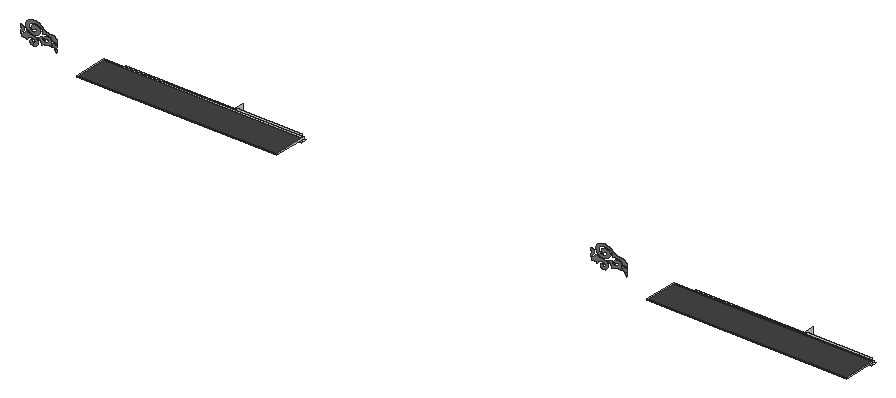
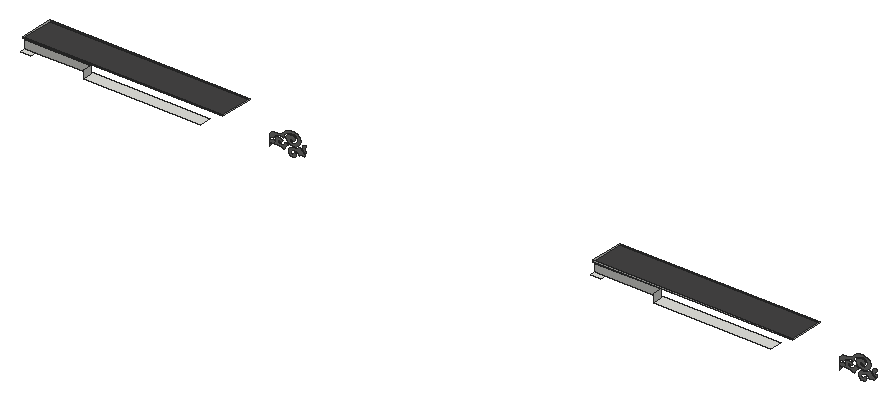
# SketchUp Ruby script. Lengths in inches.
U = 1.inch
M = Sketchup.active_model
def pt(a) = Geom::Point3d.new(a.map { |v| v * U })
def face(e, loops, mat)
  f = e.add_face(loops[0].map { |a| pt(a) })
  loops[1..].each { |l| e.add_face(l.map { |a| pt(a) }).erase! }
  f.material = f.back_material = mat if mat
  f
end
# faces: each face lists its corners as indices into pts; further lists are holes
def faces(e, pts, list, mat = nil) = list.each { |f| face(e, (f[0].is_a?(Array) ? f : [f]).map { |l| l.map { |i| pts[i] } }, mat) }
# xy, xz, yz: faces in a plane at the given z, y or x. An outline is a flat list of corners, or four numbers for a rectangle; further outlines are holes
def ring(l) = l.size == 4 ? [[l[0], l[1]], [l[2], l[1]], [l[2], l[3]], [l[0], l[3]]] : l.each_slice(2).to_a
def flat(e, list, mat, &to3) = list.each { |f| face(e, (f[0].is_a?(Array) ? f : [f]).map { |l| ring(l).map { |u, v| to3.(u, v) } }, mat) }
def xy(e, z, list, mat = nil) = flat(e, list, mat) { |x, y| [x, y, z] }
def xz(e, y, list, mat = nil) = flat(e, list, mat) { |x, z| [x, y, z] }
def yz(e, x, list, mat = nil) = flat(e, list, mat) { |y, z| [x, y, z] }
def lines(e, pts, list) = list.each { |a, b| e.add_line(pt(pts[a]), pt(pts[b])) }
# prism: a flat outline (further loops are holes) pulled along v
def prism(e, loops, v, mat = nil)
  f = face(e, loops, mat); d = Geom::Vector3d.new(v.map { |x| x * U })
  f.pushpull(f.normal.samedirection?(d) ? d.length : -d.length)
end
def box(e, o, s, mat = nil) = prism(e, [[o, [o[0] + s[0], o[1], o[2]], [o[0] + s[0], o[1] + s[1], o[2]], [o[0], o[1] + s[1], o[2]]]], [0, 0, s[2]], mat)
def at(x, y, z, deg = 0) = Geom::Transformation.translation(pt([x, y, z])) * Geom::Transformation.rotation(ORIGIN, Z_AXIS, deg.degrees)
def axes(o, x, y, z) = Geom::Transformation.new([*x, 0, *y, 0, *z, 0, *pt(o).to_a, 1])
def part(name) = M.definitions.add(name)
# library, detail: a bought-in or finely detailed component or shape, given as its bounding box
def library(name, o, s) = part(name).tap { |d| box(d.entities, o, s) }
def detail(e, o, s) = box(e.add_group.entities, o, s)
def put(e, d, t, mat = nil) = e.add_instance(d, t).tap { |i| i.material = mat if mat }
def group(e, t, mat = nil) = e.add_group.tap { |g| g.transformation = t; g.material = mat if mat }.entities
root = M.entities
M.materials.add("[0043_SaddleBrown]4").color = [124, 123, 122]
M.materials.add("[Granite Dark Gray]").color = [69, 68, 68]
xy(root,251.46,[[3079.62,589.17,3079.62,616,3336.64,616,3336.64,595.44,3457.61,595.44,3457.61,589.17],[4330.25,589.17,4330.25,616,4587.26,616,4587.26,595.44,4708.23,595.44,4708.23,589.17],[3457.61,595.44,3480.67,608.75],[4708.23,595.44,4731.3,608.75]])
xy(root,265.8125,[[3053.01,515.0625,3491.44,589.17],[4303.63,515.0625,4742.06,589.17]],"[Granite Dark Gray]")
xz(root,515.0625,[[3053.01,265.8125,3491.44,268.4375],[4303.63,265.8125,4742.06,268.4375]],"[Granite Dark Gray]")
xz(root,589.17,[[3053.01,265.8125,3491.44,268.4375],[4303.63,265.8125,4742.06,268.4375]])
xz(root,589.17,[[2899.09,240.53,2897.49,240.59,2895.9375,240.89,2894.51,241.42,2893.27,242.16,2892.27,243.07,2891.56,244.1,2891.16,245.23,2891.11,246.39,2891.17,246.75,2891.28,247.1,2891.44,247.44,2891.65,247.77,2891.91,248.09,2892.21,248.38,2892.55,248.64,2892.92,248.89,2893.33,249.1,2893.77,249.28,2894.23,249.43,2894.71,249.54,2894.79,249.03,2894.91,248.52,2895.07,248.02,2895.28,247.53,2895.52,247.05,2895.8,246.58,2896.12,246.12,2896.48,245.67,2896.87,245.24,2897.29,244.83,2897.75,244.4375,2898.24,244.07,2899.17,244.4,2900.02,244.84,2900.77,245.37,2901.4,245.97,2901.89,246.64,2902.23,247.35,2902.42,248.09,2902.44,248.85,2902.3,249.59,2902.01,250.32,2901.57,251,2900.98,251.625,2900.14,252.57,2899.07,253.38,2897.82,254.04,2896.42,254.51,2894.92,254.8,2893.37,254.88,2891.83,254.75,2890.34,254.42,2888.97,253.9,2887.76,253.2,2886.74,252.35,2885.96,251.39,2885.74,251.13,2885.54,250.86,2885.35,250.6,2885.17,250.32,2885,250.05,2884.85,249.77,2884.71,249.48,2884.58,249.2,2884.36,248.62,2884.27,248.32,2884.2,248.02,2883.51,248.6875,2882.71,249.28,2881.81,249.8,2880.83,250.24,2879.78,250.58,2878.6875,250.83,2877.55,250.97,2876.41,251.02,2875.26,250.96,2874.13,250.8,2873.04,250.54,2872,250.18,2872.22,250.49,2872.41,250.81,2872.57,251.13,2872.71,251.47,2872.83,251.8,2872.91,252.14,2872.97,252.49,2873,252.83,2873.01,253.18,2872.98,253.53,2872.93,253.875,2872.85,254.22,2874,254.84,2875.09,255.51,2876.15,256.21,2877.15,256.95,2878.11,257.73,2879.01,258.53,2879.86,259.37,2880.65,260.23,2881.38,261.12,2882.05,262.04,2882.66,262.97,2883.21,263.93,2883.82,263.15,2884.54,262.41,2885.35,261.73,2886.26,261.12,2887.25,260.57,2888.3125,260.1,2889.44,259.71,2890.61,259.41,2891.82,259.19,2893.05,259.0625,2894.29,259.03,2895.54,259.08,2897.95,258.68,2900.24,257.98,2902.32,257,2904.125,255.77,2905.61,254.34,2906.73,252.74,2907.44,251.03,2907.73,249.25,2907.58,247.46,2907.01,245.72,2906.02,244.08,2904.65,242.59,2903.52,241.76,2902.18,241.125,2900.68,240.71],[4149.72,240.53,4148.11,240.59,4146.5625,240.89,4145.14,241.42,4143.89,242.16,4142.9,243.07,4142.18,244.1,4141.79,245.23,4141.73,246.39,4141.79,246.75,4141.9,247.1,4142.07,247.44,4142.28,247.77,4142.53,248.09,4142.83,248.38,4143.17,248.64,4143.55,248.89,4143.96,249.1,4144.39,249.28,4144.85,249.43,4145.33,249.54,4145.41,249.03,4145.54,248.52,4145.7,248.02,4145.9,247.53,4146.15,247.05,4146.43,246.58,4146.75,246.12,4147.1,245.67,4147.49,245.24,4147.92,244.83,4148.375,244.4375,4148.86,244.07,4149.8,244.4,4150.65,244.84,4151.4,245.37,4152.02,245.97,4152.51,246.64,4152.86,247.35,4153.04,248.09,4153.07,248.85,4152.93,249.59,4152.64,250.32,4152.19,251,4151.6,251.625,4150.77,252.57,4149.7,253.38,4148.44,254.04,4147.04,254.51,4145.54,254.8,4143.99,254.88,4142.45,254.75,4140.97,254.42,4139.6,253.9,4138.38,253.2,4137.37,252.35,4136.58,251.39,4136.37,251.13,4136.17,250.86,4135.97,250.6,4135.79,250.32,4135.63,250.05,4135.47,249.77,4135.33,249.48,4135.21,249.2,4135.09,248.91,4134.99,248.62,4134.9,248.32,4134.83,248.02,4134.13,248.6875,4133.33,249.28,4132.44,249.8,4131.46,250.24,4130.41,250.58,4129.3125,250.83,4128.18,250.97,4127.03,251.02,4125.88,250.96,4124.75,250.8,4123.66,250.54,4122.625,250.18,4122.84,250.49,4123.03,250.81,4123.2,251.13,4123.34,251.47,4123.45,251.8,4123.54,252.14,4123.6,252.49,4123.63,252.83,4123.63,253.18,4123.61,253.53,4123.56,253.875,4123.48,254.22,4124.62,254.84,4125.72,255.51,4126.77,256.21,4127.78,256.95,4128.73,257.73,4129.63,258.53,4130.48,259.37,4131.27,260.23,4132.01,261.12,4132.68,262.04,4133.29,262.97,4133.84,263.93,4134.45,263.15,4135.16,262.41,4135.98,261.73,4136.89,261.12,4137.875,260.57,4138.9375,260.1,4140.06,259.71,4141.23,259.41,4142.44,259.19,4143.67,259.0625,4144.92,259.03,4146.16,259.08,4148.58,258.68,4150.86,257.98,4152.94,257,4154.75,255.77,4156.24,254.34,4157.35,252.74,4158.07,251.03,4158.35,249.25,4158.21,247.46,4157.63,245.72,4156.64,244.08,4155.27,242.59,4154.15,241.76,4152.8,241.125,4151.31,240.71],[2949.62,243.61,2949.34,244.05,2949.04,244.49,2948.74,244.92,2948.42,245.34,2948.09,245.77,2947.75,246.18,2947.4,246.6,2947.04,247,2946.28,247.8,2945.88,248.1875,2945.47,248.57,2945.75,248.76,2946.04,248.9375,2946.35,249.1,2946.68,249.24,2947.02,249.36,2947.37,249.47,2947.73,249.56,2948.1,249.625,2948.47,249.68,2948.85,249.71,2949.23,249.72,2949.62,249.7],[4200.24,243.61,4199.96,244.05,4199.67,244.49,4199.36,244.92,4199.05,245.34,4198.72,245.77,4198.38,246.18,4198.03,246.6,4197.29,247.4,4196.9,247.8,4196.5,248.1875,4196.1,248.57,4196.37,248.76,4196.67,248.9375,4196.98,249.1,4197.3,249.24,4197.64,249.36,4197.99,249.47,4198.35,249.56,4198.72,249.625,4199.1,249.68,4199.48,249.71,4199.86,249.72,4200.24,249.7],[2916.57,248.92,2916.46,249.99,2916.23,251.04,2915.89,252.09,2915.44,253.11,2914.89,254.1,2914.24,255.07,2913.49,255.99,2912.64,256.87,2911.71,257.7,2910.6875,258.48,2909.59,259.21,2908.42,259.87,2909.04,260.07,2910.26,260.51,2910.86,260.74,2911.45,260.97,2912.04,261.22,2912.62,261.48,2913.19,261.74,2913.75,262.01,2914.3125,262.29,2914.86,262.58,2915.4,262.88,2915.51,261.48,2916.03,260.125,2916.95,258.89,2918.23,257.82,2919.79,256.98,2921.57,256.41,2923.47,256.13,2925.42,256.15,2927.32,256.48,2929.07,257.1,2930.59,257.97,2931.81,259.07,2931.85,259.41,2931.87,259.75,2931.87,260.43,2931.81,261.11,2931.76,261.45,2931.69,261.79,2931.61,262.12,2931.52,262.46,2931.42,262.79,2931.29,263.12,2930.7,263.3,2930.07,263.42,2929.43,263.46,2928.78,263.43,2928.15,263.32,2927.55,263.15,2927,262.9,2926.5,262.6,2926.08,262.24,2925.75,261.85,2925.5,261.41,2925.36,260.96,2924.95,261.08,2924.5625,261.23,2924.18,261.39,2923.82,261.57,2923.47,261.77,2923.14,261.98,2922.83,262.2,2922.53,262.44,2922.26,262.69,2922.02,262.96,2921.79,263.23,2921.59,263.51,2922.18,264.63,2923.07,265.64,2924.23,266.5,2925.61,267.17,2927.14,267.62,2928.78,267.84,2930.4375,267.81,2932.06,267.54,2933.5625,267.03,2934.89,266.3125,2935.99,265.42,2936.81,264.375,2936.25,263.4375,2935.8,262.46,2935.48,261.47,2935.28,260.45,2935.2,259.43,2935.25,258.41,2935.43,257.39,2935.73,256.39,2936.15,255.41,2936.69,254.47,2937.35,253.56,2938.11,252.69,2936.23,252.81,2934.35,252.84,2932.46,252.8,2930.59,252.67,2928.72,252.47,2926.88,252.1875,2925.06,251.83,2923.27,251.39,2921.53,250.88,2919.82,250.3,2918.17,249.64],
  [4167.2,248.92,4167.08,249.99,4166.85,251.04,4166.51,252.09,4166.07,253.11,4165.51,254.1,4164.86,255.07,4164.11,255.99,4163.27,256.87,4162.33,257.7,4161.3125,258.48,4160.22,259.21,4159.05,259.87,4159.67,260.07,4160.89,260.51,4161.48,260.74,4162.08,260.97,4162.66,261.22,4163.24,261.48,4163.81,261.74,4164.38,262.01,4164.9375,262.29,4165.48,262.58,4166.02,262.88,4166.13,261.48,4166.66,260.125,4167.58,258.89,4168.85,257.82,4170.41,256.98,4172.19,256.41,4174.1,256.13,4176.05,256.15,4177.94,256.48,4179.69,257.1,4181.21,257.97,4182.43,259.07,4182.47,259.41,4182.49,259.75,4182.5,260.09,4182.49,260.43,4182.47,260.77,4182.43,261.11,4182.38,261.45,4182.32,261.79,4182.24,262.12,4182.15,262.46,4182.04,262.79,4181.92,263.12,4181.33,263.3,4180.7,263.42,4180.05,263.46,4179.41,263.43,4178.77,263.32,4178.17,263.15,4177.62,262.9,4177.13,262.6,4176.71,262.24,4176.37,261.85,4176.13,261.41,4175.98,260.96,4175.58,261.08,4175.1875,261.23,4174.81,261.39,4174.44,261.57,4174.09,261.77,4173.76,261.98,4173.45,262.2,4173.16,262.44,4172.89,262.69,4172.64,262.96,4172.42,263.23,4172.22,263.51,4172.8,264.63,4173.69,265.64,4174.85,266.5,4176.23,267.17,4177.77,267.62,4179.4,267.84,4181.0625,267.81,4182.68,267.54,4184.1875,267.03,4185.52,266.3125,4186.62,265.42,4187.44,264.375,4186.875,263.4375,4186.43,262.46,4186.11,261.47,4185.9,260.45,4185.83,259.43,4185.88,258.41,4186.06,257.39,4186.36,256.39,4186.78,255.41,4187.32,254.47,4187.97,253.56,4188.74,252.69,4186.86,252.81,4184.97,252.84,4183.09,252.8,4181.21,252.67,4179.35,252.47,4177.5,252.1875,4175.68,251.83,4173.9,251.39,4172.15,250.88,4170.45,250.3,4168.8,249.64],[2945.4,252.36,2944.3,252.47,2943.24,252.71,2942.24,253.0625,2941.34,253.53,2940.55,254.09,2939.89,254.73,2939.38,255.44,2939.04,256.2,2938.78,256.55,2938.625,256.93,2938.57,257.32,2938.62,257.71,2938.78,258.08,2939.03,258.43,2939.37,258.74,2939.78,258.99,2940.26,259.18,2940.78,259.31,2941.32,259.36,2941.86,259.33,2942.32,259.26,2942.78,259.16,2943.21,259.03,2943.63,258.87,2944.03,258.6875,2944.41,258.48,2944.76,258.25,2945.08,257.99,2945.36,257.72,2945.61,257.43,2945.83,257.13,2946.01,256.8125,2946.35,256.95,2946.6875,257.09,2947.02,257.24,2947.34,257.4,2947.66,257.57,2947.97,257.75,2948.27,257.93,2948.56,258.125,2948.84,258.32,2949.11,258.53,2949.37,258.74,2949.62,258.96,2949.62,253.18,2948.64,252.79,2947.6,252.53,2946.51,252.38],[4196.02,252.36,4194.92,252.47,4193.86,252.71,4192.87,253.0625,4191.96,253.53,4191.17,254.09,4190.51,254.73,4190.01,255.44,4189.66,256.2,4189.41,256.55,4189.25,256.93,4189.2,257.32,4189.25,257.71,4189.4,258.08,4189.65,258.43,4189.99,258.74,4190.41,258.99,4190.88,259.18,4191.4,259.31,4191.94,259.36,4192.48,259.33,4192.95,259.26,4193.4,259.16,4193.84,259.03,4194.26,258.87,4194.66,258.6875,4195.03,258.48,4195.38,258.25,4195.7,257.99,4195.99,257.72,4196.24,257.43,4196.45,257.13,4196.63,256.8125,4196.98,256.95,4197.3125,257.09,4197.65,257.24,4197.97,257.4,4198.28,257.57,4198.59,257.75,4198.89,257.93,4199.18,258.125,4199.46,258.32,4199.73,258.53,4199.99,258.74,4200.24,258.96,4200.24,253.18,4199.27,252.79,4198.22,252.53,4197.13,252.38],[2869.23,255.94,2869.23,260.6875,2870.31,261.02,2871.27,261.5,2872.07,262.125,2872.67,262.86,2873.04,263.66,2873.17,264.5,2873.04,265.35,2872.67,266.15,2872.07,266.88,2871.27,267.51,2870.31,267.99,2869.23,268.32,2869.23,272.35,2870.47,272.27,2871.69,272.07,2872.86,271.73,2873.93,271.26,2874.9,270.6875,2875.74,270.02,2876.42,269.26,2876.9375,268.44,2877.28,267.56,2877.43,266.67,2877.39,265.76,2877.16,264.875,2876.8125,264.01,2876.4,263.17,2875.93,262.33,2875.4,261.52,2874.81,260.73,2874.16,259.96,2873.47,259.22,2872.71,258.5,2871.91,257.8125,2871.0625,257.16,2870.17,256.53],[4119.85,255.94,4119.85,260.6875,4120.93,261.02,4121.9,261.5,4122.7,262.125,4123.3,262.86,4123.67,263.66,4123.79,264.5,4123.67,265.35,4123.3,266.15,4122.7,266.88,4121.9,267.51,4120.93,267.99,4119.85,268.32,4119.85,272.35,4121.1,272.27,4122.32,272.07,4123.48,271.73,4124.56,271.26,4125.52,270.6875,4126.36,270.02,4127.04,269.26,4127.5625,268.44,4127.9,267.56,4128.05,266.67,4128.01,265.76,4127.79,264.875,4127.4375,264.01,4127.03,263.17,4126.55,262.33,4126.02,261.52,4125.43,260.73,4124.79,259.96,4124.09,259.22,4123.34,258.5,4122.54,257.8125,4121.6875,257.16,4120.79,256.53],
  [2949.62,260.7,2949.25,261.39,2948.75,262.04,2948.13,262.64,2947.4,263.17,2946.58,263.61,2945.68,263.97,2944.71,264.24,2943.7,264.41,2942.68,264.47,2941.65,264.42,2940.63,264.28,2939.66,264.03,2939.22,265.63,2938.4,267.16,2937.24,268.56,2935.76,269.79,2934.01,270.83,2932.04,271.64,2929.91,272.19,2927.68,272.47,2925.41,272.48,2923.18,272.2,2921.04,271.65,2919.07,270.85,2919.01,272.875,2918.54,274.87,2917.68,276.79,2916.4375,278.6,2914.85,280.27,2912.93,281.75,2910.75,283.01,2908.33,284.03,2905.73,284.79,2903,285.27,2900.21,285.46,2897.41,285.35,2894.96,284.63,2892.75,283.58,2890.86,282.24,2889.36,280.66,2888.32,278.9,2887.76,277.03,2887.72,275.12,2888.1875,273.24,2889.15,271.46,2890.57,269.85,2892.4,268.46,2894.5625,267.36,2895.96,266.91,2897.45,266.68,2898.97,266.68,2900.47,266.89,2901.87,267.33,2903.12,267.96,2904.17,268.76,2904.96,269.69,2905.48,270.73,2905.69,271.82,2905.6,272.91,2905.19,273.97,2904.91,274.36,2904.54,274.7,2904.07,274.98,2903.54,275.19,2902.96,275.32,2902.36,275.37,2901.75,275.32,2901.17,275.19,2900.64,274.98,2900.18,274.7,2899.8,274.36,2899.52,273.97,2899.39,273.75,2899.23,273.53,2899.04,273.32,2898.83,273.13,2898.6,272.95,2898.35,272.78,2898.08,272.625,2897.8,272.49,2897.5,272.37,2897.18,272.27,2896.86,272.1875,2896.53,272.125,2895.95,272.37,2895.42,272.67,2894.94,273.01,2894.52,273.39,2894.16,273.8,2893.89,274.25,2893.68,274.71,2893.5625,275.1875,2893.52,275.67,2893.57,276.16,2893.69,276.64,2893.9,277.1,2894.29,277.72,2894.77,278.31,2895.33,278.86,2895.98,279.36,2896.69,279.81,2897.47,280.2,2898.3,280.52,2899.17,280.79,2900.08,280.98,2901.01,281.1,2901.95,281.15,2902.9,281.125,2904.39,280.95,2905.84,280.64,2907.22,280.19,2908.5,279.62,2909.66,278.92,2910.69,278.12,2911.55,277.23,2912.25,276.26,2912.76,275.24,2913.07,274.17,2913.1875,273.09,2913.1,272,2912.5,270.37,2911.57,268.8125,2910.35,267.37,2908.86,266.06,2907.13,264.92,2905.1875,263.97,2903.08,263.23,2900.85,262.71,2898.53,262.42,2896.1875,262.375,2893.85,262.57,2891.59,263,2889.39,264.08,2887.41,265.36,2885.67,266.82,2884.22,268.42,2883.06,270.15,2882.22,271.97,2881.71,273.85,2881.55,275.77,2881.73,277.68,2882.25,279.5625,2883.11,281.375,2884.29,283.1,2886.09,284.97,2888.31,286.6,2890.88,287.93,2893.72,288.93,2896.76,289.57,2899.9,289.83,2903.06,289.71,2906.14,289.2,2909.0625,288.32,2911.74,287.1,2914.09,285.58,2916.04,283.78,2916.58,283.04,2917.17,282.32,2917.81,281.61,2918.49,280.93,2919.22,280.27,2919.98,279.64,2920.79,279.04,2921.64,278.46,2922.52,277.91,2923.44,277.4,2924.39,276.91,2925.375,276.46,2926.68,276.01,2928.01,275.62,2929.375,275.28,2930.76,274.99,2932.17,274.76,2933.59,274.59,2935.02,274.47,2936.46,274.41,2937.9,274.41,2939.34,274.47,2940.78,274.58,2942.2,274.75,2943.32,273.47,2943.9,272.84,2944.49,272.22,2945.1,271.6,2945.71,270.99,2946.33,270.38,2947.61,269.18,2948.27,268.6,2948.9375,268.01,2949.62,267.4375],[4200.24,260.7,4199.875,261.39,4199.375,262.04,4198.76,262.64,4198.03,263.17,4197.2,263.61,4196.3,263.97,4195.34,264.24,4194.33,264.41,4193.3,264.47,4192.27,264.42,4191.26,264.28,4190.28,264.03,4189.84,265.63,4189.03,267.16,4187.86,268.56,4186.38,269.79,4184.63,270.83,4182.66,271.64,4180.53,272.19,4178.3,272.47,4176.04,272.48,4173.8,272.2,4171.67,271.65,4169.7,270.85,4169.63,272.875,4169.17,274.87,4168.3,276.79,4167.0625,278.6,4165.47,280.27,4163.56,281.75,4161.37,283.01,4158.95,284.03,4156.35,284.79,4153.63,285.27,4150.84,285.46,4148.04,285.35,4145.59,284.63,4143.37,283.58,4141.48,282.24,4139.99,280.66,4138.94,278.9,4138.39,277.03,4138.34,275.12,4138.8125,273.24,4139.78,271.46,4141.2,269.85,4143.02,268.46,4145.1875,267.36,4146.58,266.91,4148.07,266.68,4149.6,266.68,4151.09,266.89,4152.49,267.33,4153.75,267.96,4154.79,268.76,4155.59,269.69,4156.11,270.73,4156.32,271.82,4156.22,272.91,4155.81,273.97,4155.54,274.36,4155.16,274.7,4154.7,274.98,4154.16,275.19,4153.59,275.32,4152.98,275.37,4152.38,275.32,4151.8,275.19,4151.27,274.98,4150.8,274.7,4150.43,274.36,4150.15,273.97,4150.01,273.75,4149.85,273.53,4149.66,273.32,4149.45,273.13,4149.22,272.95,4148.97,272.78,4148.71,272.625,4148.42,272.49,4148.12,272.37,4147.81,272.27,4147.49,272.1875,4147.16,272.125,4146.58,272.37,4146.04,272.67,4145.56,273.01,4145.14,273.39,4144.79,273.8,4144.51,274.25,4144.31,274.71,4144.1875,275.1875,4144.15,275.67,4144.19,276.16,4144.32,276.64,4144.52,277.1,4144.91,277.72,4145.39,278.31,4145.96,278.86,4146.6,279.36,4147.32,279.81,4148.09,280.2,4148.92,280.52,4149.8,280.79,4150.7,280.98,4151.63,281.1,4152.58,281.15,4153.52,281.125,4155.02,280.95,4156.46,280.64,4157.84,280.19,4159.12,279.62,4160.29,278.92,4161.31,278.12,4162.18,277.23,4162.87,276.26,4163.38,275.24,4163.7,274.17,4163.8125,273.09,4163.73,272,4163.12,270.37,4162.2,268.8125,4160.98,267.37,4159.49,266.06,4157.75,264.92,4155.8125,263.97,4153.7,263.23,4151.47,262.71,4149.16,262.42,4146.8125,262.375,4144.48,262.57,4142.21,263,4140.02,264.08,4138.03,265.36,4136.3,266.82,4134.84,268.42,4133.68,270.15,4132.84,271.97,4132.34,273.85,4132.17,275.77,4132.35,277.68,4132.88,279.5625,4133.74,281.375,4134.91,283.1,4136.72,284.97,4138.94,286.6,4141.5,287.93,4144.35,288.93,4147.38,289.57,4150.52,289.83,4153.68,289.71,4156.77,289.2,4159.6875,288.32,4162.36,287.1,4164.71,285.58,4166.67,283.78,4167.21,283.04,4167.8,282.32,4168.43,281.61,4169.12,280.93,4169.84,280.27,4170.61,279.64,4171.42,279.04,4172.26,278.46,4173.15,277.91,4174.07,277.4,4175.02,276.91,4176,276.46,4177.3,276.01,4178.64,275.62,4180,275.28,4181.39,274.99,4182.79,274.76,4184.21,274.59,4185.65,274.47,4187.09,274.41,4188.53,274.41,4189.97,274.47,4191.4,274.58,4192.83,274.75,4193.38,274.11,4193.95,273.47,4194.53,272.84,4195.12,272.22,4195.72,271.6,4196.33,270.99,4196.96,270.38,4197.59,269.78,4198.24,269.18,4198.9,268.6,4199.5625,268.01,4200.24,267.4375]],"[0043_SaddleBrown]4")
xz(root,595.44,[[3336.64,251.46,3480.67,268.4375],[4587.26,251.46,4731.3,268.4375]])
yz(root,3053.01,[[515.0625,265.8125,589.17,268.4375]])
yz(root,3336.64,[[595.44,251.46,616,268.4375]])
yz(root,3491.44,[[515.0625,265.8125,589.17,268.4375]])
yz(root,4303.63,[[515.0625,265.8125,589.17,268.4375]])
yz(root,4587.26,[[595.44,251.46,616,268.4375]])
yz(root,4742.06,[[515.0625,265.8125,589.17,268.4375]])
